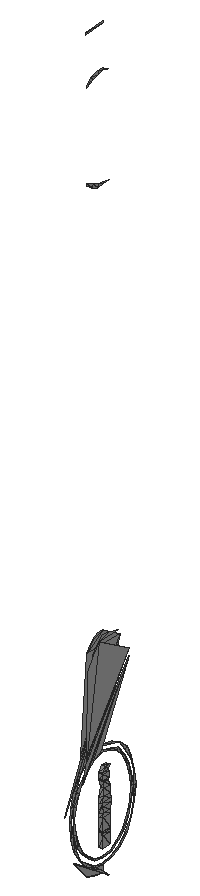
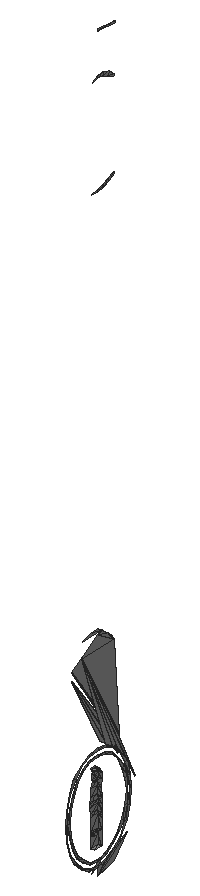
# SketchUp Ruby script. Lengths in inches.
U = 1.inch
M = Sketchup.active_model
def pt(a) = Geom::Point3d.new(a.map { |v| v * U })
def face(e, loops, mat)
  f = e.add_face(loops[0].map { |a| pt(a) })
  loops[1..].each { |l| e.add_face(l.map { |a| pt(a) }).erase! }
  f.material = f.back_material = mat if mat
  f
end
# faces: each face lists its corners as indices into pts; further lists are holes
def faces(e, pts, list, mat = nil) = list.each { |f| face(e, (f[0].is_a?(Array) ? f : [f]).map { |l| l.map { |i| pts[i] } }, mat) }
# xy, xz, yz: faces in a plane at the given z, y or x. An outline is a flat list of corners, or four numbers for a rectangle; further outlines are holes
def ring(l) = l.size == 4 ? [[l[0], l[1]], [l[2], l[1]], [l[2], l[3]], [l[0], l[3]]] : l.each_slice(2).to_a
def flat(e, list, mat, &to3) = list.each { |f| face(e, (f[0].is_a?(Array) ? f : [f]).map { |l| ring(l).map { |u, v| to3.(u, v) } }, mat) }
def xy(e, z, list, mat = nil) = flat(e, list, mat) { |x, y| [x, y, z] }
def xz(e, y, list, mat = nil) = flat(e, list, mat) { |x, z| [x, y, z] }
def yz(e, x, list, mat = nil) = flat(e, list, mat) { |y, z| [x, y, z] }
def lines(e, pts, list) = list.each { |a, b| e.add_line(pt(pts[a]), pt(pts[b])) }
# prism: a flat outline (further loops are holes) pulled along v
def prism(e, loops, v, mat = nil)
  f = face(e, loops, mat); d = Geom::Vector3d.new(v.map { |x| x * U })
  f.pushpull(f.normal.samedirection?(d) ? d.length : -d.length)
end
def box(e, o, s, mat = nil) = prism(e, [[o, [o[0] + s[0], o[1], o[2]], [o[0] + s[0], o[1] + s[1], o[2]], [o[0], o[1] + s[1], o[2]]]], [0, 0, s[2]], mat)
def at(x, y, z, deg = 0) = Geom::Transformation.translation(pt([x, y, z])) * Geom::Transformation.rotation(ORIGIN, Z_AXIS, deg.degrees)
def axes(o, x, y, z) = Geom::Transformation.new([*x, 0, *y, 0, *z, 0, *pt(o).to_a, 1])
def part(name) = M.definitions.add(name)
# library, detail: a bought-in or finely detailed component or shape, given as its bounding box
def library(name, o, s) = part(name).tap { |d| box(d.entities, o, s) }
def detail(e, o, s) = box(e.add_group.entities, o, s)
def put(e, d, t, mat = nil) = e.add_instance(d, t).tap { |i| i.material = mat if mat }
def group(e, t, mat = nil) = e.add_group.tap { |g| g.transformation = t; g.material = mat if mat }.entities
root = M.entities
M.materials.add("Material \#1").color = [140, 140, 140]
xy(root,58.189,[[263.949,328.15,263.973,328.15,263.949,328.205],[263.973,328.15,263.973,328.205,263.949,328.205]],"Material \#1")
xy(root,58.585,[[263.949,328.167,263.949,328.199,263.973,328.199],[263.949,328.167,263.973,328.199,263.973,328.167]],"Material \#1")
xz(root,328.15,[[263.949,58.189,263.973,58.253,263.973,58.189]],"Material \#1")
xz(root,328.156,[[263.949,58.476,263.973,58.513,263.973,58.476]],"Material \#1")
yz(root,263.949,[[328.177,58.122,328.125,58.131,328.127,58.14],[328.177,58.122,328.127,58.14,328.177,58.132],[328.177,58.122,328.177,58.132,328.229,58.131],[328.125,58.131,328.077,58.157,328.081,58.166],[328.125,58.131,328.081,58.166,328.127,58.14],
  [328.229,58.131,328.177,58.132,328.227,58.14],[328.229,58.131,328.227,58.14,328.277,58.157],[328.227,58.14,328.274,58.166,328.277,58.157],[328.077,58.157,328.035,58.199,328.041,58.206],[328.077,58.157,328.041,58.206,328.081,58.166],
  [328.277,58.157,328.274,58.166,328.319,58.199],[328.274,58.166,328.314,58.206,328.319,58.199],[328.035,58.199,328.004,58.254,328.01,58.259],[328.035,58.199,328.01,58.259,328.041,58.206],[328.319,58.199,328.314,58.206,328.351,58.254],
  [328.314,58.206,328.344,58.259,328.351,58.254],[328.004,58.254,327.984,58.318,327.991,58.321],[328.004,58.254,327.991,58.321,328.01,58.259],[328.351,58.254,328.344,58.259,328.371,58.318],[328.344,58.259,328.364,58.321,328.371,58.318],
  [327.984,58.318,327.977,58.387,327.984,58.387],[327.984,58.318,327.984,58.387,327.991,58.321],[328.371,58.318,328.364,58.321,328.378,58.387],[328.364,58.321,328.37,58.387,328.378,58.387],[327.977,58.387,327.984,58.455,327.991,58.453],
  [327.977,58.387,327.991,58.453,327.984,58.387],[328.37,58.387,328.364,58.453,328.371,58.455],[328.37,58.387,328.371,58.455,328.378,58.387],[327.991,58.453,327.984,58.455,328.01,58.514],[328.364,58.453,328.344,58.514,328.351,58.519],
  [328.364,58.453,328.351,58.519,328.371,58.455],[327.984,58.455,328.004,58.519,328.01,58.514],[328.01,58.514,328.004,58.519,328.041,58.567],[328.344,58.514,328.314,58.567,328.319,58.574],[328.344,58.514,328.319,58.574,328.351,58.519],
  [328.004,58.519,328.035,58.574,328.041,58.567],[328.041,58.567,328.035,58.574,328.081,58.607],[328.314,58.567,328.274,58.607,328.277,58.616],[328.314,58.567,328.277,58.616,328.319,58.574],[328.035,58.574,328.077,58.616,328.081,58.607],
  [328.081,58.607,328.077,58.616,328.127,58.633],[328.274,58.607,328.227,58.633,328.229,58.643],[328.274,58.607,328.229,58.643,328.277,58.616],[328.077,58.616,328.125,58.643,328.127,58.633],[328.127,58.633,328.125,58.643,328.177,58.642],
  [328.227,58.633,328.177,58.642,328.177,58.652],[328.227,58.633,328.177,58.652,328.229,58.643],[328.177,58.642,328.125,58.643,328.177,58.652]],"Material \#1")
yz(root,263.95,[[328.177,58.05,327.978,58.176,328.078,58.12],[328.177,58.05,328.065,58.084,327.978,58.176],[328.177,58.05,328.119,58.059,328.065,58.084],[328.177,58.05,328.078,58.12,328.126,58.097],[328.177,58.05,328.126,58.097,328.177,58.089],
  [327.924,58.431,328.029,58.667,328.288,59.173],[328.002,58.572,328.288,59.173,328.037,58.619],[328.037,58.619,328.288,59.173,328.078,58.654],[328.078,58.654,328.288,59.173,328.126,58.676],[328.029,58.667,328.032,58.673,328.288,59.173],
  [328.032,58.673,328.033,58.68,328.288,59.173],[328.033,58.68,328.034,58.6875,328.288,59.173],[328.034,58.6875,328.066,59.173,328.288,59.173],[328.066,59.173,328.088,59.202,328.115,59.224],[328.066,59.173,328.115,59.224,328.177,59.244],
  [328.066,59.173,328.177,59.244,328.288,59.173],[328.115,59.224,328.145,59.239,328.177,59.244]],"Material \#1")
yz(root,263.952,[[328.177,61.418,328.138,61.422,328.14,61.437],[328.177,61.418,328.14,61.437,328.177,61.432],[328.177,61.418,328.177,61.432,328.216,61.422],[328.138,61.422,328.101,61.436,328.105,61.45],[328.138,61.422,328.105,61.45,328.14,61.437],
  [328.101,61.436,328.067,61.457,328.073,61.47],[328.101,61.436,328.073,61.47,328.105,61.45],[328.073,61.941,328.067,61.954,328.105,61.961],[328.067,61.954,328.101,61.975,328.105,61.961],[328.105,61.961,328.101,61.975,328.14,61.974],
  [328.14,61.974,328.101,61.975,328.138,61.989],[328.14,61.974,328.138,61.989,328.177,61.978],[328.214,61.974,328.177,61.978,328.177,61.993],[328.177,61.978,328.138,61.989,328.177,61.993],[328.061,62.196,328.059,62.211,328.177,62.21],
  [328.177,62.21,328.059,62.211,328.177,62.225]],"Material \#1")
yz(root,263.955,[[328.177,58.089,328.119,58.1,328.121,58.109],[328.177,58.089,328.121,58.109,328.177,58.099],[328.177,58.089,328.177,58.099,328.235,58.1],[328.177,58.099,328.233,58.109,328.235,58.1],[328.119,58.1,328.065,58.129,328.069,58.138],
  [328.119,58.1,328.069,58.138,328.121,58.109],[328.235,58.1,328.233,58.109,328.29,58.129],[328.233,58.109,328.286,58.138,328.29,58.129],[328.065,58.129,328.018,58.177,328.023,58.184],[328.065,58.129,328.023,58.184,328.069,58.138],
  [328.29,58.129,328.286,58.138,328.336,58.177],[328.286,58.138,328.331,58.184,328.336,58.177],[328.018,58.177,327.982,58.238,327.989,58.243],[328.018,58.177,327.989,58.243,328.023,58.184],[328.336,58.177,328.331,58.184,328.372,58.238],
  [328.331,58.184,328.365,58.243,328.372,58.238],[327.982,58.238,327.96,58.31,327.967,58.3125],[327.982,58.238,327.967,58.3125,327.989,58.243],[328.372,58.238,328.365,58.243,328.394,58.31],[328.365,58.243,328.387,58.3125,328.394,58.31],
  [327.96,58.31,327.952,58.387,327.96,58.387],[327.96,58.31,327.96,58.387,327.967,58.3125],[328.394,58.31,328.387,58.3125,328.402,58.387],[328.387,58.3125,328.395,58.387,328.402,58.387],[327.952,58.387,327.96,58.464,327.967,58.461],
  [327.952,58.387,327.967,58.461,327.96,58.387],[328.395,58.387,328.387,58.461,328.394,58.464],[328.395,58.387,328.394,58.464,328.402,58.387],[327.967,58.461,327.96,58.464,327.989,58.53],[328.387,58.461,328.365,58.53,328.372,58.535],
  [328.387,58.461,328.372,58.535,328.394,58.464],[327.96,58.464,327.982,58.535,327.989,58.53],[327.989,58.53,327.982,58.535,328.023,58.59],[328.365,58.53,328.331,58.59,328.336,58.597],[328.365,58.53,328.336,58.597,328.372,58.535],
  [327.982,58.535,328.018,58.597,328.023,58.59],[328.023,58.59,328.018,58.597,328.069,58.635],[328.331,58.59,328.286,58.635,328.29,58.644],[328.331,58.59,328.29,58.644,328.336,58.597],[328.018,58.597,328.065,58.644,328.069,58.635],
  [328.069,58.635,328.065,58.644,328.121,58.664],[328.286,58.635,328.233,58.664,328.235,58.674],[328.286,58.635,328.235,58.674,328.29,58.644],[328.065,58.644,328.119,58.674,328.121,58.664],[328.121,58.664,328.119,58.674,328.177,58.674],
  [328.233,58.664,328.177,58.674,328.177,58.684],[328.233,58.664,328.177,58.684,328.235,58.674],[328.119,58.674,328.177,58.684,328.177,58.674]],"Material \#1")
yz(root,263.973,[[328.15,58.189,328.15,58.253,328.205,58.189],[328.205,58.189,328.15,58.253,328.205,58.253],[328.15,58.253,328.157,58.258,328.205,58.253],[328.205,58.253,328.157,58.258,328.198,58.258],[328.157,58.258,328.157,58.268,328.198,58.258],
  [328.198,58.258,328.157,58.268,328.198,58.268],[328.157,58.268,328.15,58.273,328.198,58.268],[328.198,58.268,328.15,58.273,328.205,58.273],[328.15,58.273,328.15,58.337,328.205,58.273],[328.205,58.273,328.15,58.337,328.205,58.337],
  [328.15,58.337,328.156,58.357,328.205,58.337],[328.205,58.337,328.156,58.357,328.199,58.357],[328.156,58.357,328.148,58.385,328.199,58.357],[328.199,58.357,328.148,58.385,328.207,58.385],[328.148,58.385,328.148,58.413,328.207,58.385],
  [328.207,58.385,328.148,58.413,328.207,58.413],[328.148,58.413,328.156,58.441,328.207,58.413],[328.207,58.413,328.156,58.441,328.199,58.441],[328.156,58.441,328.156,58.476,328.199,58.441],[328.199,58.441,328.156,58.476,328.199,58.476],
  [328.156,58.476,328.156,58.513,328.199,58.476],[328.199,58.476,328.156,58.513,328.188,58.513],[328.156,58.513,328.15,58.523,328.188,58.513],[328.188,58.513,328.15,58.523,328.194,58.523],[328.15,58.523,328.15,58.545,328.194,58.523],
  [328.194,58.523,328.15,58.545,328.194,58.545],[328.15,58.545,328.156,58.555,328.194,58.545],[328.194,58.545,328.156,58.555,328.188,58.555],[328.156,58.555,328.167,58.585,328.188,58.555],[328.188,58.555,328.167,58.585,328.199,58.585]],"Material \#1")
yz(root,263.975,[[328.177,58.05,328.126,58.097,328.078,58.12],[328.002,58.572,328.037,58.619,328.32,59.055],[328.002,58.572,328.32,59.055,328.029,58.667],[328.037,58.619,328.078,58.654,328.32,59.055],[328.078,58.654,328.126,58.676,328.32,59.055],
  [328.029,58.667,328.316,59.098,328.032,58.673],[328.032,58.673,328.316,59.098,328.033,58.68],[328.033,58.68,328.316,59.098,328.034,58.6875],[328.034,58.6875,328.316,59.098,328.035,58.695],[328.035,58.695,328.115,59.224,328.038,59.098],
  [328.035,58.695,328.316,59.098,328.115,59.224],[328.066,59.173,328.115,59.224,328.088,59.202],[328.115,59.224,328.177,59.244,328.145,59.239],[328.115,59.224,328.24,59.224,328.177,59.244]],"Material \#1")
p = [[263.949,328.15,58.189],[263.949,328.153,58.267],[263.973,328.15,58.253],[263.949,328.153,58.347],[263.949,328.152,58.371],[263.973,328.148,58.385],
  [263.973,328.148,58.385],[263.973,328.156,58.357],[263.949,328.153,58.347],[263.949,328.15,58.333],[263.949,328.153,58.347],[263.973,328.156,58.357],
  [263.949,328.153,58.267],[263.949,328.15,58.333],[263.973,328.15,58.337],[263.973,328.156,58.357],[263.973,328.15,58.337],[263.949,328.15,58.333],
  [263.973,328.15,58.337],[263.973,328.15,58.273],[263.949,328.153,58.267],[263.949,328.202,58.261],[263.973,328.198,58.268],[263.973,328.205,58.273],
  [263.949,328.153,58.267],[263.973,328.157,58.268],[263.973,328.157,58.258],[263.949,328.153,58.267],[263.973,328.15,58.253],[263.949,328.153,58.267],
  [263.973,328.15,58.273],[263.949,328.202,58.261],[263.973,328.205,58.253],[263.973,328.198,58.258],[263.949,328.202,58.261],[263.949,328.148,58.399],
  [263.949,328.152,58.427],[263.973,328.156,58.441],[263.949,328.152,58.371],[263.949,328.148,58.399],[263.973,328.148,58.413],[263.973,328.156,58.441],
  [263.973,328.148,58.413],[263.949,328.148,58.399],[263.973,328.148,58.413],[263.973,328.148,58.385],[263.949,328.152,58.371],[263.949,328.152,58.427],
  [263.949,328.156,58.476],[263.973,328.156,58.476],[263.973,328.156,58.476],[263.973,328.156,58.441],[263.949,328.152,58.427],[263.949,328.156,58.476],
  [263.949,328.153,58.518],[263.973,328.156,58.513],[263.949,328.153,58.518],[263.949,328.153,58.55],[263.973,328.15,58.545],[263.973,328.15,58.523],
  [263.949,328.153,58.55],[263.973,328.156,58.555],[263.973,328.15,58.545],[263.949,328.153,58.518],[263.973,328.15,58.523],[263.973,328.156,58.513],
  [263.949,328.191,58.55],[263.973,328.194,58.545],[263.973,328.188,58.555],[263.949,328.191,58.518],[263.973,328.188,58.513],[263.973,328.194,58.523],
  [263.949,328.153,58.55],[263.949,328.167,58.585],[263.973,328.167,58.585],[263.973,328.156,58.555],[263.949,328.153,58.55],[263.952,328.196,61.611],
  [263.952,328.117,61.761],[263.954,328.117,61.761],[263.954,328.196,61.611],[263.952,328.238,61.65],[263.952,328.252,61.622],[263.954,328.252,61.622],
  [263.954,328.238,61.65],[263.953,328.269,61.591],[263.953,328.25,61.568],[263.955,328.25,61.568],[263.955,328.269,61.591],[263.953,328.227,61.552],
  [263.955,328.227,61.552],[263.952,328.211,61.583],[263.954,328.211,61.583],[263.952,328.158,61.8],[263.954,328.158,61.8],[263.952,328.102,61.789],
  [263.954,328.102,61.789],[263.953,328.085,61.82],[263.955,328.086,61.82],[263.953,328.104,61.843],[263.955,328.104,61.843],[263.953,328.127,61.858],
  [263.955,328.127,61.858],[263.952,328.144,61.827],[263.954,328.144,61.827]]
faces(root,p,[[0,1,2],[3,4,5],[6,7,8],[9,10,11],[12,13,14],[15,16,17],[18,19,20],[21,22,23],
  [24,25,26],[27,26,28],[29,30,25],[31,32,33],[34,33,22],[35,36,37],[38,39,40],[41,42,43],
  [44,45,46],[47,48,49],[50,51,52],[53,54,55],[56,57,58],[58,59,56],[60,61,62],[63,64,65],
  [66,67,68],[69,70,71],[72,73,74],[74,75,76],[77,78,79],[79,80,77],[81,82,83],[83,84,81],
  [85,86,87],[87,88,85],[86,89,90],[90,87,86],[89,91,92],[92,90,89],[91,77,80],[80,92,91],
  [93,81,84],[84,94,93],[82,85,88],[88,83,82],[78,95,96],[96,79,78],[95,97,98],[98,96,95],
  [97,99,100],[100,98,97],[99,101,102],[102,100,99],[101,103,104],[104,102,101],[103,93,94],[94,104,103]],"Material \#1")
